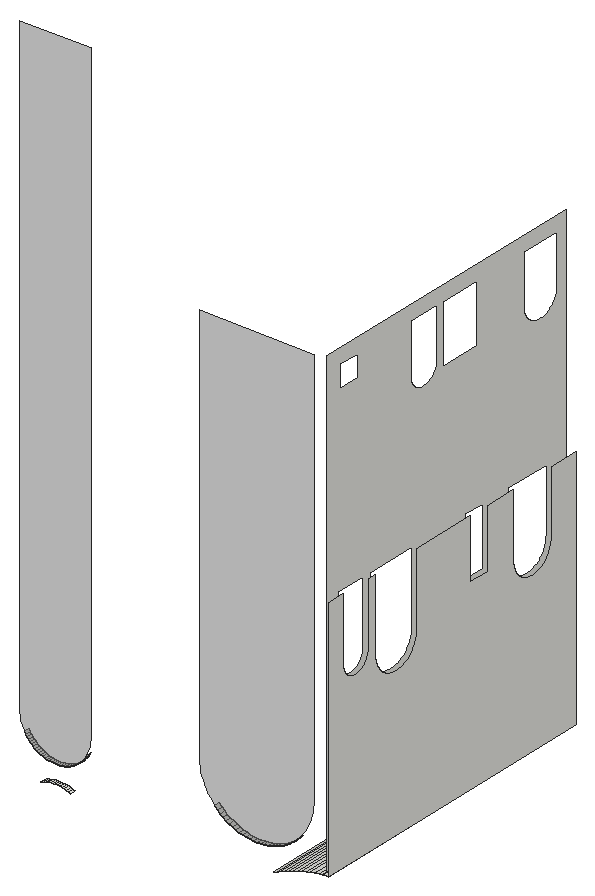
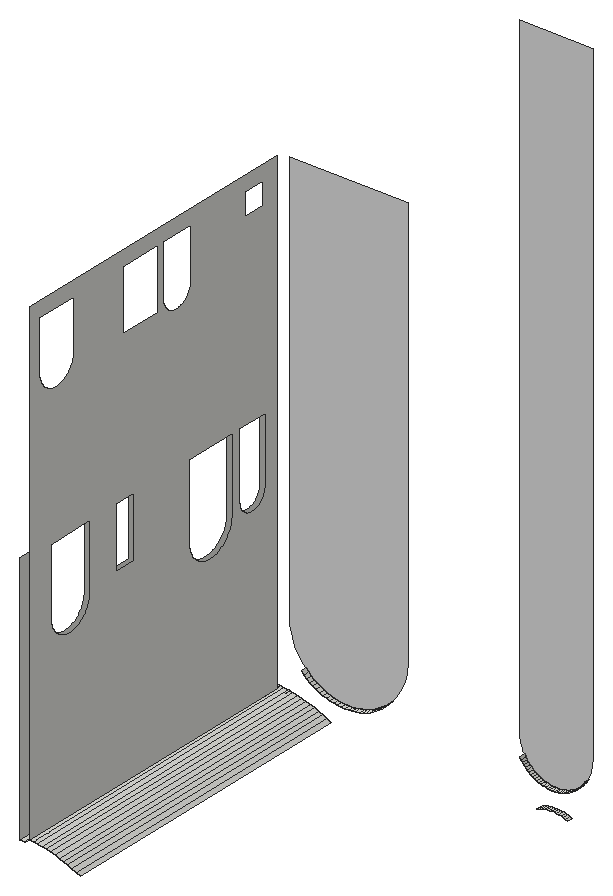
# SketchUp Ruby script. Lengths in inches.
U = 1.inch
M = Sketchup.active_model
def pt(a) = Geom::Point3d.new(a.map { |v| v * U })
def face(e, loops, mat)
  f = e.add_face(loops[0].map { |a| pt(a) })
  loops[1..].each { |l| e.add_face(l.map { |a| pt(a) }).erase! }
  f.material = f.back_material = mat if mat
  f
end
# faces: each face lists its corners as indices into pts; further lists are holes
def faces(e, pts, list, mat = nil) = list.each { |f| face(e, (f[0].is_a?(Array) ? f : [f]).map { |l| l.map { |i| pts[i] } }, mat) }
# xy, xz, yz: faces in a plane at the given z, y or x. An outline is a flat list of corners, or four numbers for a rectangle; further outlines are holes
def ring(l) = l.size == 4 ? [[l[0], l[1]], [l[2], l[1]], [l[2], l[3]], [l[0], l[3]]] : l.each_slice(2).to_a
def flat(e, list, mat, &to3) = list.each { |f| face(e, (f[0].is_a?(Array) ? f : [f]).map { |l| ring(l).map { |u, v| to3.(u, v) } }, mat) }
def xy(e, z, list, mat = nil) = flat(e, list, mat) { |x, y| [x, y, z] }
def xz(e, y, list, mat = nil) = flat(e, list, mat) { |x, z| [x, y, z] }
def yz(e, x, list, mat = nil) = flat(e, list, mat) { |y, z| [x, y, z] }
def lines(e, pts, list) = list.each { |a, b| e.add_line(pt(pts[a]), pt(pts[b])) }
# prism: a flat outline (further loops are holes) pulled along v
def prism(e, loops, v, mat = nil)
  f = face(e, loops, mat); d = Geom::Vector3d.new(v.map { |x| x * U })
  f.pushpull(f.normal.samedirection?(d) ? d.length : -d.length)
end
def box(e, o, s, mat = nil) = prism(e, [[o, [o[0] + s[0], o[1], o[2]], [o[0] + s[0], o[1] + s[1], o[2]], [o[0], o[1] + s[1], o[2]]]], [0, 0, s[2]], mat)
def at(x, y, z, deg = 0) = Geom::Transformation.translation(pt([x, y, z])) * Geom::Transformation.rotation(ORIGIN, Z_AXIS, deg.degrees)
def axes(o, x, y, z) = Geom::Transformation.new([*x, 0, *y, 0, *z, 0, *pt(o).to_a, 1])
def part(name) = M.definitions.add(name)
# library, detail: a bought-in or finely detailed component or shape, given as its bounding box
def library(name, o, s) = part(name).tap { |d| box(d.entities, o, s) }
def detail(e, o, s) = box(e.add_group.entities, o, s)
def put(e, d, t, mat = nil) = e.add_instance(d, t).tap { |i| i.material = mat if mat }
def group(e, t, mat = nil) = e.add_group.tap { |g| g.transformation = t; g.material = mat if mat }.entities
root = M.entities
M.materials.add("[Translucent Glass Gray]").color = [128, 128, 128]
M.materials["[Translucent Glass Gray]"].alpha = 0.5
xz(root,487.08,[[1771.07,263.85,1774.9375,263.97,1778.79,264.34,1782.62,264.94,1786.4,265.79,1790.12,266.87,1793.76,268.18,1797.32,269.72,1800.77,271.48,1804.1,273.45,1807.3,275.625,1810.36,278,1813.27,280.56,1816.01,283.3,1818.57,286.2,1820.94,289.26,1823.12,292.47,1825.09,295.8,1826.85,299.25,1828.39,302.8,1829.7,306.45,1830.78,310.17,1831.625,313.95,1832.23,317.77,1832.59,321.63,1832.72,325.5,1832.72,1394,1709.42,1394,1709.42,325.5,1709.54,321.63,1709.9,317.77,1710.51,313.95,1711.35,310.17,1712.43,306.45,1713.75,302.8,1715.28,299.25,1717.04,295.8,1719.01,292.47,1721.19,289.26,1723.5625,286.2,1726.125,283.3,1728.86,280.56,1731.77,278,1734.83,275.625,1738.03,273.45,1741.37,271.48,1744.82,269.72,1748.37,268.18,1752.02,266.87,1755.73,265.79,1759.51,264.94,1763.34,264.34,1767.2,263.97],[2118.63,264.71,2124.87,264.9,2131.09,265.49,2137.27,266.47,2143.36,267.83,2149.37,269.57,2155.24,271.69,2160.98,274.17,2166.55,277.01,2171.93,280.19,2177.09,283.7,2182.03,287.53,2186.72,291.67,2191.14,296.08,2195.27,300.77,2199.1,305.71,2202.61,310.88,2205.79,316.26,2208.63,321.82,2211.11,327.56,2213.23,333.4375,2214.97,339.4375,2216.34,345.54,2217.3125,351.71,2217.9,357.93,2218.1,364.18,2218.1,1054,2019.16,1054,2019.16,364.18,2019.35,357.93,2019.94,351.71,2020.92,345.54,2022.28,339.4375,2024.02,333.4375,2026.14,327.56,2028.62,321.82,2031.46,316.26,2034.64,310.88,2038.15,305.71,2041.98,300.77,2046.12,296.08,2050.53,291.67,2055.22,287.53,2060.16,283.7,2065.33,280.19,2070.71,277.01,2076.27,274.17,2082.01,271.69,2087.89,269.57,2093.89,267.83,2099.99,266.47,2106.16,265.49,2112.38,264.9]],"[Translucent Glass Gray]")
yz(root,2233.1,[[[496.08,254.8125,1012.08,1054],[633.74,509.34,636.6,509.43,639.45,509.7,642.28,510.15,645.07,510.78,647.82,511.57,650.51,512.54,653.14,513.68,655.69,514.98,658.16,516.4375,660.53,518.05,662.79,519.8,664.9375,521.7,666.96,523.72,668.86,525.87,670.61,528.13,672.22,530.5,673.68,532.96,674.98,535.52,676.11,538.14,677.08,540.84,677.88,543.59,678.51,546.38,678.96,549.21,679.23,552.0625,679.32,554.92,679.32,678.55,588.16,678.55,588.16,554.92,588.25,552.0625,588.52,549.21,588.96,546.38,589.59,543.59,590.39,540.84,591.36,538.14,592.49,535.52,593.79,532.96,595.25,530.5,596.86,528.13,598.62,525.87,600.51,523.72,602.53,521.7,604.68,519.8,606.94,518.05,609.3125,516.4375,611.78,514.98,614.33,513.68,616.96,512.54,619.65,511.57,622.4,510.78,625.19,510.15,628.02,509.7,630.875,509.43],[927.82,528.05,930.42,528.14,933.02,528.38,935.59,528.79,938.14,529.36,940.64,530.09,943.09,530.97,945.49,532,947.81,533.1875,950.05,534.51,952.21,535.98,954.27,537.58,956.22,539.3,958.07,541.15,959.79,543.1,961.39,545.16,962.86,547.32,964.18,549.5625,965.37,551.88,966.4,554.28,966.63,554.92,967.28,556.73,968.01,559.23,968.58,561.78,968.99,564.35,969.23,566.95,969.32,569.55,969.32,678.55,886.32,678.55,886.32,569.55,886.4,566.95,886.64,564.35,887.05,561.78,887.62,559.23,888.35,556.73,889,554.92,889.23,554.28,890.27,551.88,891.45,549.5625,892.78,547.32,894.24,545.16,895.84,543.1,897.5625,541.15,899.41,539.3,901.36,537.58,903.42,535.98,905.58,534.51,907.82,533.1875,910.15,532,912.54,530.97,914.99,530.09,917.5,529.36,920.04,528.79,922.61,528.38,925.21,528.14],[956.24,909.7,958.54,909.77,960.82,909.98,963.08,910.34,965.32,910.84,967.52,911.48,969.68,912.26,971.78,913.17,973.83,914.21,975.8,915.38,977.7,916.67,979.51,918.07,981.23,919.59,982.85,921.21,984.37,922.93,985.77,924.74,987.0625,926.64,988.23,928.61,989.27,930.66,990.18,932.76,990.96,934.92,991.6,937.12,992.1,939.36,992.46,941.62,992.67,943.9,992.74,946.2,992.74,1029.2,919.74,1029.2,919.74,946.2,919.82,943.9,920.03,941.62,920.39,939.36,920.89,937.12,921.53,934.92,922.31,932.76,923.22,930.66,924.26,928.61,925.43,926.64,926.71,924.74,928.12,922.93,929.64,921.21,931.26,919.59,932.98,918.07,934.79,916.67,936.6875,915.38,938.66,914.21,940.7,913.17,942.81,912.26,944.96,911.48,947.17,910.84,949.4,910.34,951.67,909.98,953.95,909.77],[745.0625,928.39,818.41,1029.2],[546.33,542.05,548.05,542.11,549.77,542.27,551.48,542.54,553.17,542.92,554.82,543.4,556.45,543.99,558.04,544.67,559.58,545.46,561.0625,546.33,562.49,547.31,563.86,548.36,565.15,549.51,566.375,550.73,567.52,552.02,568.57,553.39,569.55,554.82,569.61,554.92,570.43,556.31,571.21,557.84,571.9,559.43,572.48,561.06,572.96,562.71,573.34,564.4,573.61,566.11,573.77,567.83,573.83,569.55,573.83,678.55,518.83,678.55,518.83,569.55,518.88,567.83,519.04,566.11,519.3125,564.4,519.69,562.71,520.17,561.06,520.76,559.43,521.44,557.84,522.23,556.31,523.05,554.92,523.11,554.82,524.08,553.39,525.14,552.02,526.28,550.73,527.5,549.51,528.8,548.36,530.16,547.31,531.59,546.33,533.08,545.46,534.62,544.67,536.2,543.99,537.83,543.4,539.49,542.92,541.17,542.54,542.88,542.27,544.6,542.11],[704.59,915.82,706.18,915.86,707.77,915.99,709.35,916.2,710.91,916.5,712.46,916.875,713.98,917.34,715.48,917.88,716.95,918.5,718.375,919.2,719.77,919.98,721.12,920.83,722.42,921.75,723.67,922.73,724.86,923.79,726,924.9,727.07,926.08,728.08,927.31,729.03,928.59,729.9,929.92,730.7,931.3,731.43,932.72,732.08,934.17,732.65,935.66,733.14,937.17,733.55,938.71,733.55,1029.2,675.625,1029.2,675.625,938.71,676.04,937.17,676.53,935.66,677.1,934.17,677.75,932.72,678.47,931.3,679.28,929.92,680.15,928.59,681.09,927.31,682.1,926.08,683.18,924.9,684.32,923.79,685.51,922.73,686.76,921.75,688.0625,920.83,689.41,919.98,690.8,919.2,692.23,918.5,693.7,917.88,695.19,917.34,696.72,916.875,698.27,916.5,699.83,916.2,701.41,915.99,703,915.86],[793.72,576.55,831.72,678.55],[523.83,991.35,561.87,1029.2]]])
yz(root,2242.1,[[487.08,255.64,1021.08,255.64,1021.08,678.55,969.32,678.55,969.32,569.55,969.23,566.95,968.99,564.35,968.58,561.78,968.01,559.23,967.28,556.73,966.63,554.92,966.4,554.28,965.37,551.88,964.18,549.5625,962.86,547.32,961.39,545.16,959.79,543.1,958.07,541.15,956.22,539.3,954.27,537.58,952.21,535.98,950.05,534.51,947.81,533.1875,945.49,532,943.09,530.97,940.64,530.09,938.14,529.36,935.59,528.79,933.02,528.38,930.42,528.14,927.82,528.05,925.21,528.14,922.61,528.38,920.04,528.79,917.5,529.36,914.99,530.09,912.54,530.97,910.15,532,907.82,533.1875,905.58,534.51,903.42,535.98,901.36,537.58,899.41,539.3,897.5625,541.15,895.84,543.1,894.24,545.16,892.78,547.32,891.45,549.5625,890.27,551.88,889.23,554.28,889,554.92,888.35,556.73,887.62,559.23,887.05,561.78,886.64,564.35,886.4,566.95,886.32,569.55,886.32,678.55,831.72,678.55,831.72,576.55,793.72,576.55,793.72,678.55,679.32,678.55,679.32,554.92,679.23,552.0625,678.96,549.21,678.51,546.38,677.88,543.59,677.08,540.84,676.11,538.14,674.98,535.52,673.68,532.96,672.22,530.5,670.61,528.13,668.86,525.87,666.96,523.72,664.9375,521.7,662.79,519.8,660.53,518.05,658.16,516.4375,655.69,514.98,653.14,513.68,650.51,512.54,647.82,511.57,645.07,510.78,642.28,510.15,639.45,509.7,636.6,509.43,633.74,509.34,630.875,509.43,628.02,509.7,625.19,510.15,622.4,510.78,619.65,511.57,616.96,512.54,614.33,513.68,611.78,514.98,609.3125,516.4375,606.94,518.05,604.68,519.8,602.53,521.7,600.51,523.72,598.62,525.87,596.86,528.13,595.25,530.5,593.79,532.96,592.49,535.52,591.36,538.14,590.39,540.84,589.59,543.59,588.96,546.38,588.52,549.21,588.25,552.0625,588.16,554.92,588.16,678.55,573.83,678.55,573.83,569.55,573.77,567.83,573.61,566.11,573.34,564.4,572.96,562.71,572.48,561.06,571.9,559.43,571.21,557.84,570.43,556.31,569.61,554.92,569.55,554.82,568.57,553.39,567.52,552.02,566.375,550.73,565.15,549.51,563.86,548.36,562.49,547.31,561.0625,546.33,559.58,545.46,558.04,544.67,556.45,543.99,554.82,543.4,553.17,542.92,551.48,542.54,549.77,542.27,548.05,542.11,546.33,542.05,544.6,542.11,542.88,542.27,541.17,542.54,539.49,542.92,537.83,543.4,536.2,543.99,534.62,544.67,533.08,545.46,531.59,546.33,530.16,547.31,528.8,548.36,527.5,549.51,526.28,550.73,525.14,552.02,524.08,553.39,523.11,554.82,523.05,554.92,522.23,556.31,521.44,557.84,520.76,559.43,520.17,561.06,519.69,562.71,519.3125,564.4,519.04,566.11,518.88,567.83,518.83,569.55,518.83,678.55,487.08,678.55]])
p = [[1748.37,487.08,228.63],[1744.82,487.08,227.1],[1744.82,496.08,227.1],[1748.37,496.08,228.63],[1797.32,487.08,227.1],[1793.76,487.08,228.63],
  [1793.76,496.08,228.63],[1797.32,496.08,227.1],[1752.02,487.08,229.95],[1752.02,496.08,229.95],[1790.12,487.08,229.95],[1790.12,496.08,229.95],
  [2155.27,487.08,232.64],[2148.53,487.08,229.29],[2148.53,1012.08,229.29],[2155.27,1012.08,232.64],[1755.73,487.08,231.03],[1755.73,496.08,231.03],
  [1786.4,487.08,231.03],[1786.4,496.08,231.03],[1759.51,487.08,231.87],[1759.51,496.08,231.87],[1782.62,487.08,231.87],[1782.62,496.08,231.87],
  [1763.34,487.08,232.48],[1763.34,496.08,232.48],[1778.79,487.08,232.48],[1778.79,496.08,232.48],[1767.2,487.08,232.84],[1767.2,496.08,232.84],
  [1774.9375,487.08,232.84],[1774.9375,496.08,232.84],[2162.11,487.08,235.79],[2162.11,1012.08,235.79],[1771.07,487.08,232.96],[1771.07,496.08,232.96],
  [2169.05,487.08,238.72],[2169.05,1012.08,238.72],[2176.07,487.08,241.43],[2176.07,1012.08,241.43],[2183.18,487.08,243.92],[2183.18,1012.08,243.92],
  [2190.36,487.08,246.19],[2190.36,1012.08,246.19],[2197.6,487.08,248.23],[2197.6,1012.08,248.23],[2204.91,487.08,250.04],[2204.91,1012.08,250.04],
  [2212.27,487.08,251.63],[2212.27,1012.08,251.63],[2218.1,487.08,252.69],[2218.1,1012.08,252.69],[2219.68,1012.08,252.98],[2219.68,487.08,252.98],
  [2227.12,1012.08,254.1],[2227.12,487.08,254.1],[2233.1,1012.08,254.8125],[2233.1,496.08,254.8125],[2233.1,487.08,254.8125],[2234.6,487.08,254.99],
  [2233.1,1021.08,254.8125],[2234.6,1021.08,254.99],[2242.1,487.08,255.64],[2242.1,1021.08,255.64],[1767.2,487.08,263.97],[1771.07,487.08,263.85],
  [1771.07,496.08,263.85],[1767.2,496.08,263.97],[1774.9375,487.08,263.97],[1774.9375,496.08,263.97],[1763.34,487.08,264.34],[1763.34,496.08,264.34],
  [1778.79,487.08,264.34],[1778.79,496.08,264.34],[1759.51,487.08,264.94],[1759.51,496.08,264.94],[1782.62,487.08,264.94],[1782.62,496.08,264.94],
  [2112.38,487.08,264.9],[2118.63,487.08,264.71],[2118.63,496.08,264.71],[2112.38,496.08,264.9],[2124.87,487.08,264.9],[2124.87,496.08,264.9],
  [1755.73,487.08,265.79],[1755.73,496.08,265.79],[1786.4,487.08,265.79],[1786.4,496.08,265.79],[2106.16,487.08,265.49],[2106.16,496.08,265.49],
  [2131.09,487.08,265.49],[2131.09,496.08,265.49],[2099.99,487.08,266.47],[2099.99,496.08,266.47],[2137.27,487.08,266.47],[2137.27,496.08,266.47],
  [1752.02,487.08,266.87],[1752.02,496.08,266.87],[1790.12,487.08,266.87],[1790.12,496.08,266.87],[2093.89,487.08,267.83],[2093.89,496.08,267.83],
  [2143.36,487.08,267.83],[2143.36,496.08,267.83],[1748.37,487.08,268.18],[1748.37,496.08,268.18],[1793.76,487.08,268.18],[1793.76,496.08,268.18],
  [2087.89,487.08,269.57],[2087.89,496.08,269.57],[2149.37,487.08,269.57],[2149.37,496.08,269.57],[1744.82,487.08,269.72],[1744.82,496.08,269.72],
  [1797.32,487.08,269.72],[1797.32,496.08,269.72],[2082.01,487.08,271.69],[2082.01,496.08,271.69],[2155.24,487.08,271.69],[2155.24,496.08,271.69],
  [1741.37,487.08,271.48],[1741.37,496.08,271.48],[1800.77,487.08,271.48],[1800.77,496.08,271.48],[1738.03,487.08,273.45],[1738.03,496.08,273.45],
  [1804.1,487.08,273.45],[1804.1,496.08,273.45],[2076.27,487.08,274.17],[2076.27,496.08,274.17],[2160.98,487.08,274.17],[2160.98,496.08,274.17],
  [1734.83,487.08,275.625],[1734.83,496.08,275.625],[1807.3,487.08,275.625],[1807.3,496.08,275.625],[2070.71,487.08,277.01],[2070.71,496.08,277.01],
  [2166.55,487.08,277.01],[2166.55,496.08,277.01],[1731.77,487.08,278],[1731.77,496.08,278],[1810.36,487.08,278],[1810.36,496.08,278],
  [2065.33,487.08,280.19],[2065.33,496.08,280.19],[2171.93,487.08,280.19],[2171.93,496.08,280.19],[1728.86,487.08,280.56],[1728.86,496.08,280.56],
  [1813.27,487.08,280.56],[1813.27,496.08,280.56],[2060.16,487.08,283.7],[2060.16,496.08,283.7],[2177.09,487.08,283.7],[2177.09,496.08,283.7],
  [1726.125,487.08,283.3],[1726.125,496.08,283.3],[1816.01,487.08,283.3],[1816.01,496.08,283.3],[1723.5625,487.08,286.2],[1723.5625,496.08,286.2],
  [1818.57,487.08,286.2],[1818.57,496.08,286.2],[2055.22,487.08,287.53],[2055.22,496.08,287.53],[2182.03,487.08,287.53],[2182.03,496.08,287.53],
  [1721.19,487.08,289.26],[1721.19,496.08,289.26],[1820.94,487.08,289.26],[1820.94,496.08,289.26],[2050.53,487.08,291.67],[2050.53,496.08,291.67],
  [2186.72,487.08,291.67],[2186.72,496.08,291.67],[1719.01,487.08,292.47],[1719.01,496.08,292.47],[1823.12,487.08,292.47],[1823.12,496.08,292.47],
  [2046.12,487.08,296.08],[2046.12,496.08,296.08],[2191.14,487.08,296.08],[2191.14,496.08,296.08],[1717.04,487.08,295.8],[1717.04,496.08,295.8],
  [1825.09,487.08,295.8],[1825.09,496.08,295.8],[2218.1,496.08,252.69]]
faces(root,p,[[0,1,2,3],[4,5,6,7],[8,0,3,9],[5,10,11,6],[12,13,14,15],[16,8,9,17],[10,18,19,11],[20,16,17,21],
  [18,22,23,19],[24,20,21,25],[22,26,27,23],[28,24,25,29],[26,30,31,27],[32,12,15,33],[34,28,29,35],[30,34,35,31],
  [36,32,33,37],[38,36,37,39],[40,38,39,41],[42,40,41,43],[44,42,43,45],[46,44,45,47],[48,46,47,49],[50,48,49,51,52,53],
  [53,52,54,55],[55,54,56,57,58],[59,58,57,56,60,61],[62,59,61,63],[64,65,66,67],[65,68,69,66],[70,64,67,71],[68,72,73,69],
  [74,70,71,75],[72,76,77,73],[78,79,80,81],[79,82,83,80],[84,74,75,85],[76,86,87,77],[88,78,81,89],[82,90,91,83],
  [92,88,89,93],[90,94,95,91],[96,84,85,97],[86,98,99,87],[100,92,93,101],[94,102,103,95],[104,96,97,105],[98,106,107,99],
  [108,100,101,109],[102,110,111,103],[112,104,105,113],[106,114,115,107],[116,108,109,117],[110,118,119,111],[120,112,113,121],[114,122,123,115],
  [124,120,121,125],[122,126,127,123],[128,116,117,129],[118,130,131,119],[132,124,125,133],[126,134,135,127],[136,128,129,137],[130,138,139,131],
  [140,132,133,141],[134,142,143,135],[144,136,137,145],[138,146,147,139],[148,140,141,149],[142,150,151,143],[152,144,145,153],[146,154,155,147],
  [156,148,149,157],[150,158,159,151],[160,156,157,161],[158,162,163,159],[164,152,153,165],[154,166,167,155],[168,160,161,169],[162,170,171,163],
  [172,164,165,173],[166,174,175,167],[176,168,169,177],[170,178,179,171],[180,172,173,181],[174,182,183,175],[184,176,177,185],[178,186,187,179]])
lines(root,p,[[50,188]])
